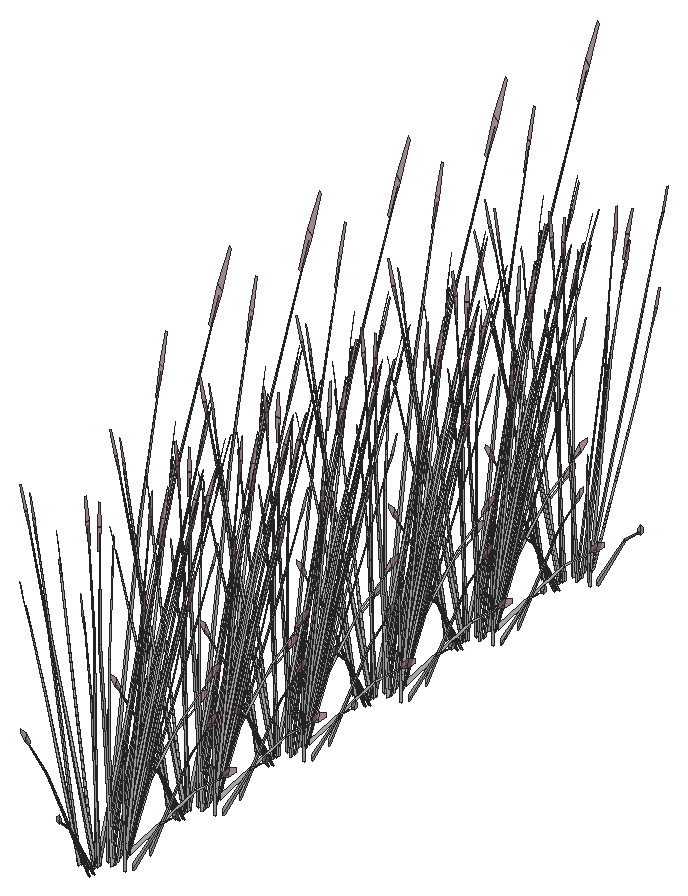
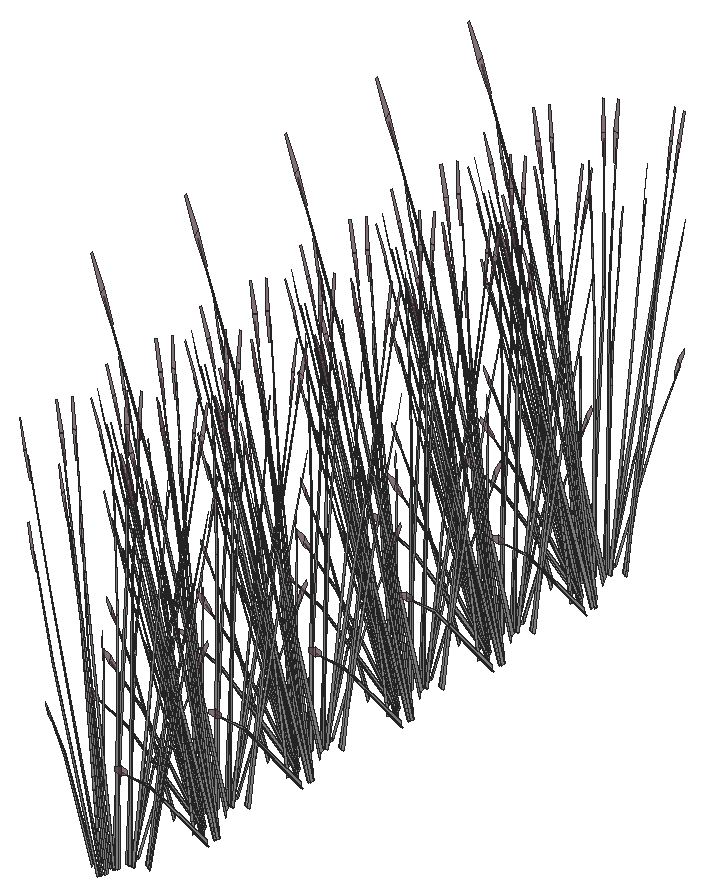
# SketchUp Ruby script. Lengths in inches.
U = 1.inch
M = Sketchup.active_model
def pt(a) = Geom::Point3d.new(a.map { |v| v * U })
def face(e, loops, mat)
  f = e.add_face(loops[0].map { |a| pt(a) })
  loops[1..].each { |l| e.add_face(l.map { |a| pt(a) }).erase! }
  f.material = f.back_material = mat if mat
  f
end
# faces: each face lists its corners as indices into pts; further lists are holes
def faces(e, pts, list, mat = nil) = list.each { |f| face(e, (f[0].is_a?(Array) ? f : [f]).map { |l| l.map { |i| pts[i] } }, mat) }
# xy, xz, yz: faces in a plane at the given z, y or x. An outline is a flat list of corners, or four numbers for a rectangle; further outlines are holes
def ring(l) = l.size == 4 ? [[l[0], l[1]], [l[2], l[1]], [l[2], l[3]], [l[0], l[3]]] : l.each_slice(2).to_a
def flat(e, list, mat, &to3) = list.each { |f| face(e, (f[0].is_a?(Array) ? f : [f]).map { |l| ring(l).map { |u, v| to3.(u, v) } }, mat) }
def xy(e, z, list, mat = nil) = flat(e, list, mat) { |x, y| [x, y, z] }
def xz(e, y, list, mat = nil) = flat(e, list, mat) { |x, z| [x, y, z] }
def yz(e, x, list, mat = nil) = flat(e, list, mat) { |y, z| [x, y, z] }
def lines(e, pts, list) = list.each { |a, b| e.add_line(pt(pts[a]), pt(pts[b])) }
# prism: a flat outline (further loops are holes) pulled along v
def prism(e, loops, v, mat = nil)
  f = face(e, loops, mat); d = Geom::Vector3d.new(v.map { |x| x * U })
  f.pushpull(f.normal.samedirection?(d) ? d.length : -d.length)
end
def box(e, o, s, mat = nil) = prism(e, [[o, [o[0] + s[0], o[1], o[2]], [o[0] + s[0], o[1] + s[1], o[2]], [o[0], o[1] + s[1], o[2]]]], [0, 0, s[2]], mat)
def at(x, y, z, deg = 0) = Geom::Transformation.translation(pt([x, y, z])) * Geom::Transformation.rotation(ORIGIN, Z_AXIS, deg.degrees)
def axes(o, x, y, z) = Geom::Transformation.new([*x, 0, *y, 0, *z, 0, *pt(o).to_a, 1])
def part(name) = M.definitions.add(name)
# library, detail: a bought-in or finely detailed component or shape, given as its bounding box
def library(name, o, s) = part(name).tap { |d| box(d.entities, o, s) }
def detail(e, o, s) = box(e.add_group.entities, o, s)
def put(e, d, t, mat = nil) = e.add_instance(d, t).tap { |i| i.material = mat if mat }
def group(e, t, mat = nil) = e.add_group.tap { |g| g.transformation = t; g.material = mat if mat }.entities
root = M.entities
M.materials.add("LightPink_Translucent").color = [144, 107, 117]
M.materials["LightPink_Translucent"].alpha = 0.75
M.materials.add("[_0053_Ivory_]").color = [200, 200, 200]
c1 = part("blade")
p = [[2.15,0.21,22],[0,0.17,0],[0.09,0.45,0],[2.18,0.31,22],[2.29,0.31,22],[0.38,0.45,0],
  [2.48,0.24,33],[2.49,0.24,33],[2.48,0.22,33]]
faces(c1.entities,p,[[0,1,2,3],[4,5,2,3],[6,3,4,7],[8,0,3,6]])
c2 = part("seeds")
p = [[0.3,-0.1,1.38],[-0.01,-0.03,1.59],[-0.01,-0.03,0.03],[0.14,-0.07,-0.07],[0.29,-0.03,3],[0.15,0.01,3.11]]
faces(c2.entities,p,[[0,1,2,3],[1,0,4,5]],"LightPink_Translucent")
c3 = part("blade with seeds")
put(c3.entities,c1,at(0,0,0))
put(c3.entities,c2,axes([2.4,0.25,30.99],[1.5799,-0.05474,1.17369],[-0.12525,1.92788,0.29478],[-0.07173,-0.02425,1.56792]))
put(root,c3,axes([680.31,309.62,38.7],[-0.1831,0.48359,0.35414],[-0.53419,-0.14105,-0.4572],[-0.04898,-0.1947,0.87481]),"[_0053_Ivory_]")
put(root,c3,axes([679.33,257.15,38.72],[-0.59846,-0.1644,0.53283],[0.20464,-0.54049,0.43934],[0.03596,0.21255,1.10256]),"[_0053_Ivory_]")
put(root,c3,axes([679.33,268.3,38.72],[-0.59846,-0.1644,0.53283],[0.20464,-0.54049,0.43934],[0.03596,0.21255,1.10256]),"[_0053_Ivory_]")
put(root,c3,axes([679.33,279.29,38.72],[-0.59846,-0.1644,0.53283],[0.20464,-0.54049,0.43934],[0.03596,0.21255,1.10256]),"[_0053_Ivory_]")
put(root,c3,axes([679.33,291.34,38.72],[-0.59846,-0.1644,0.53283],[0.20464,-0.54049,0.43934],[0.03596,0.21255,1.10256]),"[_0053_Ivory_]")
put(root,c3,axes([679.33,302.71,38.72],[-0.59846,-0.1644,0.53283],[0.20464,-0.54049,0.43934],[0.03596,0.21255,1.10256]),"[_0053_Ivory_]")
put(root,c3,axes([679.18,257.2,38.38],[-0.44753,0.21372,0.0643],[-0.21905,-0.38973,0.50621],[0.04322,0.1718,0.77189]),"[_0053_Ivory_]")
put(root,c3,axes([679.18,268.34,38.38],[-0.44753,0.21372,0.0643],[-0.21905,-0.38973,0.50621],[0.04322,0.1718,0.77189]),"[_0053_Ivory_]")
put(root,c3,axes([679.18,279.34,38.38],[-0.44753,0.21372,0.0643],[-0.21905,-0.38973,0.50621],[0.04322,0.1718,0.77189]),"[_0053_Ivory_]")
put(root,c3,axes([679.18,291.38,38.38],[-0.44753,0.21372,0.0643],[-0.21905,-0.38973,0.50621],[0.04322,0.1718,0.77189]),"[_0053_Ivory_]")
put(root,c3,axes([679.18,302.75,38.38],[-0.44753,0.21372,0.0643],[-0.21905,-0.38973,0.50621],[0.04322,0.1718,0.77189]),"[_0053_Ivory_]")
put(root,c3,axes([680.48,251.65,38.38],[0.44753,-0.21372,0.0643],[0.21905,0.38973,0.50621],[-0.04322,-0.1718,0.77189]),"[_0053_Ivory_]")
put(root,c3,axes([680.48,262.8,38.38],[0.44753,-0.21372,0.0643],[0.21905,0.38973,0.50621],[-0.04322,-0.1718,0.77189]),"[_0053_Ivory_]")
put(root,c3,axes([680.48,273.79,38.38],[0.44753,-0.21372,0.0643],[0.21905,0.38973,0.50621],[-0.04322,-0.1718,0.77189]),"[_0053_Ivory_]")
put(root,c3,axes([680.48,285.84,38.38],[0.44753,-0.21372,0.0643],[0.21905,0.38973,0.50621],[-0.04322,-0.1718,0.77189]),"[_0053_Ivory_]")
put(root,c3,axes([680.48,297.2,38.38],[0.44753,-0.21372,0.0643],[0.21905,0.38973,0.50621],[-0.04322,-0.1718,0.77189]),"[_0053_Ivory_]")
put(root,c3,axes([680.48,309.18,38.38],[0.44753,-0.21372,0.0643],[0.21905,0.38973,0.50621],[-0.04322,-0.1718,0.77189]),"[_0053_Ivory_]")
put(root,c3,axes([679.02,258.125,38.37],[0.07699,0.10127,1.74944],[0.6213,0.03978,-0.27667],[0.06248,0.22333,0.14031]),"[_0053_Ivory_]")
put(root,c3,axes([679.02,269.27,38.37],[0.07699,0.10127,1.74944],[0.6213,0.03978,-0.27667],[0.06248,0.22333,0.14031]),"[_0053_Ivory_]")
put(root,c3,axes([679.02,280.26,38.37],[0.07699,0.10127,1.74944],[0.6213,0.03978,-0.27667],[0.06248,0.22333,0.14031]),"[_0053_Ivory_]")
put(root,c3,axes([679.02,292.31,38.37],[0.07699,0.10127,1.74944],[0.6213,0.03978,-0.27667],[0.06248,0.22333,0.14031]),"[_0053_Ivory_]")
put(root,c3,axes([679.02,303.67,38.37],[0.07699,0.10127,1.74944],[0.6213,0.03978,-0.27667],[0.06248,0.22333,0.14031]),"[_0053_Ivory_]")
put(root,c3,axes([680.32,251.7,38.39],[0.59846,0.1644,0.48003],[-0.20464,0.54049,0.3958],[-0.03596,-0.21255,0.9933]),"[_0053_Ivory_]")
put(root,c3,axes([680.32,262.84,38.39],[0.59846,0.1644,0.48003],[-0.20464,0.54049,0.3958],[-0.03596,-0.21255,0.9933]),"[_0053_Ivory_]")
put(root,c3,axes([680.32,273.83,38.39],[0.59846,0.1644,0.48003],[-0.20464,0.54049,0.3958],[-0.03596,-0.21255,0.9933]),"[_0053_Ivory_]")
put(root,c3,axes([680.32,285.88,38.39],[0.59846,0.1644,0.48003],[-0.20464,0.54049,0.3958],[-0.03596,-0.21255,0.9933]),"[_0053_Ivory_]")
put(root,c3,axes([680.32,297.25,38.39],[0.59846,0.1644,0.48003],[-0.20464,0.54049,0.3958],[-0.03596,-0.21255,0.9933]),"[_0053_Ivory_]")
put(root,c3,axes([680.32,309.22,38.39],[0.59846,0.1644,0.48003],[-0.20464,0.54049,0.3958],[-0.03596,-0.21255,0.9933]),"[_0053_Ivory_]")
put(root,c3,axes([679.34,256.76,38.7],[0.1831,-0.48359,0.35414],[0.53419,0.14105,-0.4572],[0.04898,0.1947,0.87481]),"[_0053_Ivory_]")
put(root,c3,axes([679.34,267.91,38.7],[0.1831,-0.48359,0.35414],[0.53419,0.14105,-0.4572],[0.04898,0.1947,0.87481]),"[_0053_Ivory_]")
put(root,c3,axes([679.34,278.9,38.7],[0.1831,-0.48359,0.35414],[0.53419,0.14105,-0.4572],[0.04898,0.1947,0.87481]),"[_0053_Ivory_]")
put(root,c3,axes([679.34,290.94,38.7],[0.1831,-0.48359,0.35414],[0.53419,0.14105,-0.4572],[0.04898,0.1947,0.87481]),"[_0053_Ivory_]")
put(root,c3,axes([679.34,302.31,38.7],[0.1831,-0.48359,0.35414],[0.53419,0.14105,-0.4572],[0.04898,0.1947,0.87481]),"[_0053_Ivory_]")
put(root,c3,axes([680.06,258.48,39.3],[0.4197,-0.36076,-0.06488],[0.38456,0.39511,-0.29416],[0.02707,0.11196,0.97024]),"[_0053_Ivory_]")
put(root,c3,axes([680.06,269.63,39.3],[0.4197,-0.36076,-0.06488],[0.38456,0.39511,-0.29416],[0.02707,0.11196,0.97024]),"[_0053_Ivory_]")
put(root,c3,axes([680.06,280.62,39.3],[0.4197,-0.36076,-0.06488],[0.38456,0.39511,-0.29416],[0.02707,0.11196,0.97024]),"[_0053_Ivory_]")
put(root,c3,axes([680.06,292.67,39.3],[0.4197,-0.36076,-0.06488],[0.38456,0.39511,-0.29416],[0.02707,0.11196,0.97024]),"[_0053_Ivory_]")
put(root,c3,axes([680.06,304.03,39.3],[0.4197,-0.36076,-0.06488],[0.38456,0.39511,-0.29416],[0.02707,0.11196,0.97024]),"[_0053_Ivory_]")
put(root,c3,axes([679.16,256.96,38.6875],[0.59433,-0.29278,-0.1216],[0.29207,0.51964,-0.67495],[0.07842,0.21898,1.02557]),"[_0053_Ivory_]")
put(root,c3,axes([679.16,268.11,38.6875],[0.59433,-0.29278,-0.1216],[0.29207,0.51964,-0.67495],[0.07842,0.21898,1.02557]),"[_0053_Ivory_]")
put(root,c3,axes([679.16,279.1,38.6875],[0.59433,-0.29278,-0.1216],[0.29207,0.51964,-0.67495],[0.07842,0.21898,1.02557]),"[_0053_Ivory_]")
put(root,c3,axes([679.16,291.14,38.6875],[0.59433,-0.29278,-0.1216],[0.29207,0.51964,-0.67495],[0.07842,0.21898,1.02557]),"[_0053_Ivory_]")
put(root,c3,axes([679.16,302.51,38.6875],[0.59433,-0.29278,-0.1216],[0.29207,0.51964,-0.67495],[0.07842,0.21898,1.02557]),"[_0053_Ivory_]")
put(root,c3,axes([682.2,251.16,38.36],[-0.06168,0.04803,1.77383],[-0.60432,-0.16205,-0.16761],[-0.02188,-0.20961,0.31391]),"[_0053_Ivory_]")
put(root,c3,axes([682.2,262.31,38.36],[-0.06168,0.04803,1.77383],[-0.60432,-0.16205,-0.16761],[-0.02188,-0.20961,0.31391]),"[_0053_Ivory_]")
put(root,c3,axes([682.2,273.3,38.36],[-0.06168,0.04803,1.77383],[-0.60432,-0.16205,-0.16761],[-0.02188,-0.20961,0.31391]),"[_0053_Ivory_]")
put(root,c3,axes([682.2,285.34,38.36],[-0.06168,0.04803,1.77383],[-0.60432,-0.16205,-0.16761],[-0.02188,-0.20961,0.31391]),"[_0053_Ivory_]")
put(root,c3,axes([682.2,296.71,38.36],[-0.06168,0.04803,1.77383],[-0.60432,-0.16205,-0.16761],[-0.02188,-0.20961,0.31391]),"[_0053_Ivory_]")
put(root,c3,axes([682.2,308.6875,38.36],[-0.06168,0.04803,1.77383],[-0.60432,-0.16205,-0.16761],[-0.02188,-0.20961,0.31391]),"[_0053_Ivory_]")
put(root,c3,axes([681.72,252.55,38.6875],[-0.6675,-0.03116,-0.1216],[0.01824,-0.58993,-0.67495],[0.04637,-0.2272,1.02557]),"[_0053_Ivory_]")
put(root,c3,axes([681.72,263.69,38.6875],[-0.6675,-0.03116,-0.1216],[0.01824,-0.58993,-0.67495],[0.04637,-0.2272,1.02557]),"[_0053_Ivory_]")
put(root,c3,axes([681.72,274.6875,38.6875],[-0.6675,-0.03116,-0.1216],[0.01824,-0.58993,-0.67495],[0.04637,-0.2272,1.02557]),"[_0053_Ivory_]")
put(root,c3,axes([681.72,286.73,38.6875],[-0.6675,-0.03116,-0.1216],[0.01824,-0.58993,-0.67495],[0.04637,-0.2272,1.02557]),"[_0053_Ivory_]")
put(root,c3,axes([681.72,298.1,38.6875],[-0.6675,-0.03116,-0.1216],[0.01824,-0.58993,-0.67495],[0.04637,-0.2272,1.02557]),"[_0053_Ivory_]")
put(root,c3,axes([681.72,310.07,38.6875],[-0.6675,-0.03116,-0.1216],[0.01824,-0.58993,-0.67495],[0.04637,-0.2272,1.02557]),"[_0053_Ivory_]")
put(root,c3,axes([681.46,252.64,38.7],[-0.41095,0.33109,0.35414],[-0.38901,-0.37805,-0.4572],[0.05919,-0.19208,0.87481]),"[_0053_Ivory_]")
put(root,c3,axes([681.46,263.79,38.7],[-0.41095,0.33109,0.35414],[-0.38901,-0.37805,-0.4572],[0.05919,-0.19208,0.87481]),"[_0053_Ivory_]")
put(root,c3,axes([681.46,274.78,38.7],[-0.41095,0.33109,0.35414],[-0.38901,-0.37805,-0.4572],[0.05919,-0.19208,0.87481]),"[_0053_Ivory_]")
put(root,c3,axes([681.46,286.82,38.7],[-0.41095,0.33109,0.35414],[-0.38901,-0.37805,-0.4572],[0.05919,-0.19208,0.87481]),"[_0053_Ivory_]")
put(root,c3,axes([681.46,298.1875,38.7],[-0.41095,0.33109,0.35414],[-0.38901,-0.37805,-0.4572],[0.05919,-0.19208,0.87481]),"[_0053_Ivory_]")
put(root,c3,axes([681.46,310.17,38.7],[-0.41095,0.33109,0.35414],[-0.38901,-0.37805,-0.4572],[0.05919,-0.19208,0.87481]),"[_0053_Ivory_]")
put(root,c3,axes([680.82,257.02,38.39],[-0.60408,0.14432,0.48003],[-0.10484,-0.56611,0.3958],[0.14207,0.16684,0.9933]),"[_0053_Ivory_]")
put(root,c3,axes([680.82,268.17,38.39],[-0.60408,0.14432,0.48003],[-0.10484,-0.56611,0.3958],[0.14207,0.16684,0.9933]),"[_0053_Ivory_]")
put(root,c3,axes([680.82,279.16,38.39],[-0.60408,0.14432,0.48003],[-0.10484,-0.56611,0.3958],[0.14207,0.16684,0.9933]),"[_0053_Ivory_]")
put(root,c3,axes([680.82,291.21,38.39],[-0.60408,0.14432,0.48003],[-0.10484,-0.56611,0.3958],[0.14207,0.16684,0.9933]),"[_0053_Ivory_]")
put(root,c3,axes([680.82,302.58,38.39],[-0.60408,0.14432,0.48003],[-0.10484,-0.56611,0.3958],[0.14207,0.16684,0.9933]),"[_0053_Ivory_]")
put(root,c3,axes([680.71,257.14,38.38],[-0.27604,0.39948,0.0643],[-0.39309,-0.23258,0.50621],[0.12709,0.12808,0.77189]),"[_0053_Ivory_]")
put(root,c3,axes([680.71,268.28,38.38],[-0.27604,0.39948,0.0643],[-0.39309,-0.23258,0.50621],[0.12709,0.12808,0.77189]),"[_0053_Ivory_]")
put(root,c3,axes([680.71,279.28,38.38],[-0.27604,0.39948,0.0643],[-0.39309,-0.23258,0.50621],[0.12709,0.12808,0.77189]),"[_0053_Ivory_]")
put(root,c3,axes([680.71,291.32,38.38],[-0.27604,0.39948,0.0643],[-0.39309,-0.23258,0.50621],[0.12709,0.12808,0.77189]),"[_0053_Ivory_]")
put(root,c3,axes([680.71,302.6875,38.38],[-0.27604,0.39948,0.0643],[-0.39309,-0.23258,0.50621],[0.12709,0.12808,0.77189]),"[_0053_Ivory_]")
put(root,c3,axes([680.625,256.68,38.7],[-0.0938,-0.50652,0.35414],[0.53623,-0.13375,-0.4572],[0.14403,0.14515,0.87481]),"[_0053_Ivory_]")
put(root,c3,axes([680.625,267.83,38.7],[-0.0938,-0.50652,0.35414],[0.53623,-0.13375,-0.4572],[0.14403,0.14515,0.87481]),"[_0053_Ivory_]")
put(root,c3,axes([680.625,278.82,38.7],[-0.0938,-0.50652,0.35414],[0.53623,-0.13375,-0.4572],[0.14403,0.14515,0.87481]),"[_0053_Ivory_]")
put(root,c3,axes([680.625,290.86,38.7],[-0.0938,-0.50652,0.35414],[0.53623,-0.13375,-0.4572],[0.14403,0.14515,0.87481]),"[_0053_Ivory_]")
put(root,c3,axes([680.625,302.23,38.7],[-0.0938,-0.50652,0.35414],[0.53623,-0.13375,-0.4572],[0.14403,0.14515,0.87481]),"[_0053_Ivory_]")
put(root,c3,axes([680.98,253.76,38.13],[-0.52482,-0.32674,1.38283],[0.55416,-0.50872,0.59665],[0.16933,0.30658,1.33663]),"[_0053_Ivory_]")
put(root,c3,axes([680.98,264.91,38.13],[-0.52482,-0.32674,1.38283],[0.55416,-0.50872,0.59665],[0.16933,0.30658,1.33663]),"[_0053_Ivory_]")
put(root,c3,axes([680.98,275.9,38.13],[-0.52482,-0.32674,1.38283],[0.55416,-0.50872,0.59665],[0.16933,0.30658,1.33663]),"[_0053_Ivory_]")
put(root,c3,axes([680.98,287.95,38.13],[-0.52482,-0.32674,1.38283],[0.55416,-0.50872,0.59665],[0.16933,0.30658,1.33663]),"[_0053_Ivory_]")
put(root,c3,axes([680.98,299.3125,38.13],[-0.52482,-0.32674,1.38283],[0.55416,-0.50872,0.59665],[0.16933,0.30658,1.33663]),"[_0053_Ivory_]")
put(root,c3,axes([680.1,257.39,38.36],[0.0018,-0.07613,1.77383],[0.52048,-0.3359,-0.16761],[0.18079,0.11989,0.31391]),"[_0053_Ivory_]")
put(root,c3,axes([680.1,268.53,38.36],[0.0018,-0.07613,1.77383],[0.52048,-0.3359,-0.16761],[0.18079,0.11989,0.31391]),"[_0053_Ivory_]")
put(root,c3,axes([680.1,279.53,38.36],[0.0018,-0.07613,1.77383],[0.52048,-0.3359,-0.16761],[0.18079,0.11989,0.31391]),"[_0053_Ivory_]")
put(root,c3,axes([680.1,291.57,38.36],[0.0018,-0.07613,1.77383],[0.52048,-0.3359,-0.16761],[0.18079,0.11989,0.31391]),"[_0053_Ivory_]")
put(root,c3,axes([680.1,302.9375,38.36],[0.0018,-0.07613,1.77383],[0.52048,-0.3359,-0.16761],[0.18079,0.11989,0.31391]),"[_0053_Ivory_]")
put(root,c3,axes([681.84,252.34,38.38],[0.49911,0.0293,0.0643],[-0.01368,0.44245,0.50621],[0.05223,-0.16948,0.77189]),"[_0053_Ivory_]")
put(root,c3,axes([681.84,263.49,38.38],[0.49911,0.0293,0.0643],[-0.01368,0.44245,0.50621],[0.05223,-0.16948,0.77189]),"[_0053_Ivory_]")
put(root,c3,axes([681.84,274.48,38.38],[0.49911,0.0293,0.0643],[-0.01368,0.44245,0.50621],[0.05223,-0.16948,0.77189]),"[_0053_Ivory_]")
put(root,c3,axes([681.84,286.52,38.38],[0.49911,0.0293,0.0643],[-0.01368,0.44245,0.50621],[0.05223,-0.16948,0.77189]),"[_0053_Ivory_]")
put(root,c3,axes([681.84,297.89,38.38],[0.49911,0.0293,0.0643],[-0.01368,0.44245,0.50621],[0.05223,-0.16948,0.77189]),"[_0053_Ivory_]")
put(root,c3,axes([681.84,309.86,38.38],[0.49911,0.0293,0.0643],[-0.01368,0.44245,0.50621],[0.05223,-0.16948,0.77189]),"[_0053_Ivory_]")
put(root,c3,axes([682.33,251.61,38.37],[-0.00586,-0.12516,1.74944],[-0.49517,-0.36172,-0.27667],[0.07656,-0.21927,0.14031]),"[_0053_Ivory_]")
put(root,c3,axes([682.33,262.76,38.37],[-0.00586,-0.12516,1.74944],[-0.49517,-0.36172,-0.27667],[0.07656,-0.21927,0.14031]),"[_0053_Ivory_]")
put(root,c3,axes([682.33,273.75,38.37],[-0.00586,-0.12516,1.74944],[-0.49517,-0.36172,-0.27667],[0.07656,-0.21927,0.14031]),"[_0053_Ivory_]")
put(root,c3,axes([682.33,285.79,38.37],[-0.00586,-0.12516,1.74944],[-0.49517,-0.36172,-0.27667],[0.07656,-0.21927,0.14031]),"[_0053_Ivory_]")
put(root,c3,axes([682.33,297.16,38.37],[-0.00586,-0.12516,1.74944],[-0.49517,-0.36172,-0.27667],[0.07656,-0.21927,0.14031]),"[_0053_Ivory_]")
put(root,c3,axes([682.33,309.14,38.37],[-0.00586,-0.12516,1.74944],[-0.49517,-0.36172,-0.27667],[0.07656,-0.21927,0.14031]),"[_0053_Ivory_]")
put(root,c3,axes([681.68,252.3,38.39],[0.43249,0.42907,0.48003],[-0.45929,0.37004,0.3958],[0.07978,-0.2013,0.9933]),"[_0053_Ivory_]")
put(root,c3,axes([681.68,263.44,38.39],[0.43249,0.42907,0.48003],[-0.45929,0.37004,0.3958],[0.07978,-0.2013,0.9933]),"[_0053_Ivory_]")
put(root,c3,axes([681.68,274.4375,38.39],[0.43249,0.42907,0.48003],[-0.45929,0.37004,0.3958],[0.07978,-0.2013,0.9933]),"[_0053_Ivory_]")
put(root,c3,axes([681.68,286.48,38.39],[0.43249,0.42907,0.48003],[-0.45929,0.37004,0.3958],[0.07978,-0.2013,0.9933]),"[_0053_Ivory_]")
put(root,c3,axes([681.68,297.85,38.39],[0.43249,0.42907,0.48003],[-0.45929,0.37004,0.3958],[0.07978,-0.2013,0.9933]),"[_0053_Ivory_]")
put(root,c3,axes([681.68,309.82,38.39],[0.43249,0.42907,0.48003],[-0.45929,0.37004,0.3958],[0.07978,-0.2013,0.9933]),"[_0053_Ivory_]")
put(root,c3,axes([682.18,253.66,38.7],[-0.52868,0.08987,0.35414],[-0.1396,-0.51376,-0.4572],[0.1515,-0.13799,0.87481]),"[_0053_Ivory_]")
put(root,c3,axes([682.18,264.81,38.7],[-0.52868,0.08987,0.35414],[-0.1396,-0.51376,-0.4572],[0.1515,-0.13799,0.87481]),"[_0053_Ivory_]")
put(root,c3,axes([682.18,275.8,38.7],[-0.52868,0.08987,0.35414],[-0.1396,-0.51376,-0.4572],[0.1515,-0.13799,0.87481]),"[_0053_Ivory_]")
put(root,c3,axes([682.18,287.84,38.7],[-0.52868,0.08987,0.35414],[-0.1396,-0.51376,-0.4572],[0.1515,-0.13799,0.87481]),"[_0053_Ivory_]")
put(root,c3,axes([682.18,299.21,38.7],[-0.52868,0.08987,0.35414],[-0.1396,-0.51376,-0.4572],[0.1515,-0.13799,0.87481]),"[_0053_Ivory_]")
put(root,c3,axes([682.18,311.1875,38.7],[-0.52868,0.08987,0.35414],[-0.1396,-0.51376,-0.4572],[0.1515,-0.13799,0.87481]),"[_0053_Ivory_]")
put(root,c3,axes([680.57,256.9375,38.6875],[0.36191,-0.53827,-0.1216],[0.52412,0.3101,-0.67495],[0.18219,0.15207,1.02557]),"[_0053_Ivory_]")
put(root,c3,axes([680.57,268.09,38.6875],[0.36191,-0.53827,-0.1216],[0.52412,0.3101,-0.67495],[0.18219,0.15207,1.02557]),"[_0053_Ivory_]")
put(root,c3,axes([680.57,279.08,38.6875],[0.36191,-0.53827,-0.1216],[0.52412,0.3101,-0.67495],[0.18219,0.15207,1.02557]),"[_0053_Ivory_]")
put(root,c3,axes([680.57,291.12,38.6875],[0.36191,-0.53827,-0.1216],[0.52412,0.3101,-0.67495],[0.18219,0.15207,1.02557]),"[_0053_Ivory_]")
put(root,c3,axes([680.57,302.49,38.6875],[0.36191,-0.53827,-0.1216],[0.52412,0.3101,-0.67495],[0.18219,0.15207,1.02557]),"[_0053_Ivory_]")
put(root,c3,axes([682.45,253.71,38.6875],[-0.56181,-0.34675,-0.1216],[0.32367,-0.50216,-0.67495],[0.15873,-0.17455,1.02557]),"[_0053_Ivory_]")
put(root,c3,axes([682.45,264.86,38.6875],[-0.56181,-0.34675,-0.1216],[0.32367,-0.50216,-0.67495],[0.15873,-0.17455,1.02557]),"[_0053_Ivory_]")
put(root,c3,axes([682.45,275.85,38.6875],[-0.56181,-0.34675,-0.1216],[0.32367,-0.50216,-0.67495],[0.15873,-0.17455,1.02557]),"[_0053_Ivory_]")
put(root,c3,axes([682.45,287.89,38.6875],[-0.56181,-0.34675,-0.1216],[0.32367,-0.50216,-0.67495],[0.15873,-0.17455,1.02557]),"[_0053_Ivory_]")
put(root,c3,axes([682.45,299.26,38.6875],[-0.56181,-0.34675,-0.1216],[0.32367,-0.50216,-0.67495],[0.15873,-0.17455,1.02557]),"[_0053_Ivory_]")
put(root,c3,axes([682.45,311.24,38.6875],[-0.56181,-0.34675,-0.1216],[0.32367,-0.50216,-0.67495],[0.15873,-0.17455,1.02557]),"[_0053_Ivory_]")
put(root,c3,axes([681.69,255.99,38.7],[-0.34557,-0.39372,0.35414],[0.39459,-0.37271,-0.4572],[0.20048,0.05671,0.87481]),"[_0053_Ivory_]")
put(root,c3,axes([681.69,267.14,38.7],[-0.34557,-0.39372,0.35414],[0.39459,-0.37271,-0.4572],[0.20048,0.05671,0.87481]),"[_0053_Ivory_]")
put(root,c3,axes([681.69,278.13,38.7],[-0.34557,-0.39372,0.35414],[0.39459,-0.37271,-0.4572],[0.20048,0.05671,0.87481]),"[_0053_Ivory_]")
put(root,c3,axes([681.69,290.18,38.7],[-0.34557,-0.39372,0.35414],[0.39459,-0.37271,-0.4572],[0.20048,0.05671,0.87481]),"[_0053_Ivory_]")
put(root,c3,axes([681.69,301.54,38.7],[-0.34557,-0.39372,0.35414],[0.39459,-0.37271,-0.4572],[0.20048,0.05671,0.87481]),"[_0053_Ivory_]")
put(root,c3,axes([682.01,256.35,38.38],[-0.03058,0.47819,0.0643],[-0.4618,-0.01311,0.50621],[0.1769,0.05004,0.77189]),"[_0053_Ivory_]")
put(root,c3,axes([682.01,267.5,38.38],[-0.03058,0.47819,0.0643],[-0.4618,-0.01311,0.50621],[0.1769,0.05004,0.77189]),"[_0053_Ivory_]")
put(root,c3,axes([682.01,278.49,38.38],[-0.03058,0.47819,0.0643],[-0.4618,-0.01311,0.50621],[0.1769,0.05004,0.77189]),"[_0053_Ivory_]")
put(root,c3,axes([682.01,290.53,38.38],[-0.03058,0.47819,0.0643],[-0.4618,-0.01311,0.50621],[0.1769,0.05004,0.77189]),"[_0053_Ivory_]")
put(root,c3,axes([682.01,301.9,38.38],[-0.03058,0.47819,0.0643],[-0.4618,-0.01311,0.50621],[0.1769,0.05004,0.77189]),"[_0053_Ivory_]")
put(root,c3,axes([682.05,256.2,38.39],[-0.44783,0.41436,0.48003],[-0.38623,-0.44004,0.3958],[0.21011,0.07643,0.9933]),"[_0053_Ivory_]")
put(root,c3,axes([682.05,267.35,38.39],[-0.44783,0.41436,0.48003],[-0.38623,-0.44004,0.3958],[0.21011,0.07643,0.9933]),"[_0053_Ivory_]")
put(root,c3,axes([682.05,278.34,38.39],[-0.44783,0.41436,0.48003],[-0.38623,-0.44004,0.3958],[0.21011,0.07643,0.9933]),"[_0053_Ivory_]")
put(root,c3,axes([682.05,290.38,38.39],[-0.44783,0.41436,0.48003],[-0.38623,-0.44004,0.3958],[0.21011,0.07643,0.9933]),"[_0053_Ivory_]")
put(root,c3,axes([682.05,301.75,38.39],[-0.44783,0.41436,0.48003],[-0.38623,-0.44004,0.3958],[0.21011,0.07643,0.9933]),"[_0053_Ivory_]")
put(root,c3,axes([682.26,254.89,38.7],[-0.50475,-0.17543,0.35414],[0.14722,-0.5118,-0.4572],[0.20322,-0.04693,0.87481]),"[_0053_Ivory_]")
put(root,c3,axes([682.26,266.04,38.7],[-0.50475,-0.17543,0.35414],[0.14722,-0.5118,-0.4572],[0.20322,-0.04693,0.87481]),"[_0053_Ivory_]")
put(root,c3,axes([682.26,277.03,38.7],[-0.50475,-0.17543,0.35414],[0.14722,-0.5118,-0.4572],[0.20322,-0.04693,0.87481]),"[_0053_Ivory_]")
put(root,c3,axes([682.26,289.07,38.7],[-0.50475,-0.17543,0.35414],[0.14722,-0.5118,-0.4572],[0.20322,-0.04693,0.87481]),"[_0053_Ivory_]")
put(root,c3,axes([682.26,300.44,38.7],[-0.50475,-0.17543,0.35414],[0.14722,-0.5118,-0.4572],[0.20322,-0.04693,0.87481]),"[_0053_Ivory_]")
put(root,c3,axes([682.26,312.42,38.7],[-0.50475,-0.17543,0.35414],[0.14722,-0.5118,-0.4572],[0.20322,-0.04693,0.87481]),"[_0053_Ivory_]")
put(root,c3,axes([682.66,253.58,38.38],[0.41695,0.26447,0.0643],[-0.24275,0.37662,0.50621],[0.13368,-0.12176,0.77189]),"[_0053_Ivory_]")
put(root,c3,axes([682.66,264.73,38.38],[0.41695,0.26447,0.0643],[-0.24275,0.37662,0.50621],[0.13368,-0.12176,0.77189]),"[_0053_Ivory_]")
put(root,c3,axes([682.66,275.72,38.38],[0.41695,0.26447,0.0643],[-0.24275,0.37662,0.50621],[0.13368,-0.12176,0.77189]),"[_0053_Ivory_]")
put(root,c3,axes([682.66,287.76,38.38],[0.41695,0.26447,0.0643],[-0.24275,0.37662,0.50621],[0.13368,-0.12176,0.77189]),"[_0053_Ivory_]")
put(root,c3,axes([682.66,299.13,38.38],[0.41695,0.26447,0.0643],[-0.24275,0.37662,0.50621],[0.13368,-0.12176,0.77189]),"[_0053_Ivory_]")
put(root,c3,axes([682.66,311.11,38.38],[0.41695,0.26447,0.0643],[-0.24275,0.37662,0.50621],[0.13368,-0.12176,0.77189]),"[_0053_Ivory_]")
put(root,c3,axes([682.54,253.47,38.39],[0.15063,0.57876,0.48003],[-0.59087,0.10045,0.3958],[0.17414,-0.13612,0.9933]),"[_0053_Ivory_]")
put(root,c3,axes([682.54,264.62,38.39],[0.15063,0.57876,0.48003],[-0.59087,0.10045,0.3958],[0.17414,-0.13612,0.9933]),"[_0053_Ivory_]")
put(root,c3,axes([682.54,275.61,38.39],[0.15063,0.57876,0.48003],[-0.59087,0.10045,0.3958],[0.17414,-0.13612,0.9933]),"[_0053_Ivory_]")
put(root,c3,axes([682.54,287.65,38.39],[0.15063,0.57876,0.48003],[-0.59087,0.10045,0.3958],[0.17414,-0.13612,0.9933]),"[_0053_Ivory_]")
put(root,c3,axes([682.54,299.02,38.39],[0.15063,0.57876,0.48003],[-0.59087,0.10045,0.3958],[0.17414,-0.13612,0.9933]),"[_0053_Ivory_]")
put(root,c3,axes([682.54,311,38.39],[0.15063,0.57876,0.48003],[-0.59087,0.10045,0.3958],[0.17414,-0.13612,0.9933]),"[_0053_Ivory_]")
put(root,c3,axes([683.83,253.56,38.36],[-0.07933,-0.00478,1.77383],[-0.32942,-0.51175,-0.16761],[0.13229,-0.16826,0.31391]),"[_0053_Ivory_]")
put(root,c3,axes([683.83,264.71,38.36],[-0.07933,-0.00478,1.77383],[-0.32942,-0.51175,-0.16761],[0.13229,-0.16826,0.31391]),"[_0053_Ivory_]")
put(root,c3,axes([683.83,275.7,38.36],[-0.07933,-0.00478,1.77383],[-0.32942,-0.51175,-0.16761],[0.13229,-0.16826,0.31391]),"[_0053_Ivory_]")
put(root,c3,axes([683.83,287.74,38.36],[-0.07933,-0.00478,1.77383],[-0.32942,-0.51175,-0.16761],[0.13229,-0.16826,0.31391]),"[_0053_Ivory_]")
put(root,c3,axes([683.83,299.11,38.36],[-0.07933,-0.00478,1.77383],[-0.32942,-0.51175,-0.16761],[0.13229,-0.16826,0.31391]),"[_0053_Ivory_]")
put(root,c3,axes([683.83,311.09,38.36],[-0.07933,-0.00478,1.77383],[-0.32942,-0.51175,-0.16761],[0.13229,-0.16826,0.31391]),"[_0053_Ivory_]")
put(root,c3,axes([682.72,255.05,38.38],[0.22307,0.42878,0.0643],[-0.40677,0.20987,0.50621],[0.17931,-0.04141,0.77189]),"[_0053_Ivory_]")
put(root,c3,axes([682.72,266.2,38.38],[0.22307,0.42878,0.0643],[-0.40677,0.20987,0.50621],[0.17931,-0.04141,0.77189]),"[_0053_Ivory_]")
put(root,c3,axes([682.72,277.1875,38.38],[0.22307,0.42878,0.0643],[-0.40677,0.20987,0.50621],[0.17931,-0.04141,0.77189]),"[_0053_Ivory_]")
put(root,c3,axes([682.72,289.23,38.38],[0.22307,0.42878,0.0643],[-0.40677,0.20987,0.50621],[0.17931,-0.04141,0.77189]),"[_0053_Ivory_]")
put(root,c3,axes([682.72,300.6,38.38],[0.22307,0.42878,0.0643],[-0.40677,0.20987,0.50621],[0.17931,-0.04141,0.77189]),"[_0053_Ivory_]")
put(root,c3,axes([682.72,312.58,38.38],[0.22307,0.42878,0.0643],[-0.40677,0.20987,0.50621],[0.17931,-0.04141,0.77189]),"[_0053_Ivory_]")
put(root,c3,axes([681.79,256.24,38.6875],[0.03252,-0.63953,-0.1216],[0.61574,0.01748,-0.67495],[0.23714,0.04442,1.02557]),"[_0053_Ivory_]")
put(root,c3,axes([681.79,267.39,38.6875],[0.03252,-0.63953,-0.1216],[0.61574,0.01748,-0.67495],[0.23714,0.04442,1.02557]),"[_0053_Ivory_]")
put(root,c3,axes([681.79,278.38,38.6875],[0.03252,-0.63953,-0.1216],[0.61574,0.01748,-0.67495],[0.23714,0.04442,1.02557]),"[_0053_Ivory_]")
put(root,c3,axes([681.79,290.43,38.6875],[0.03252,-0.63953,-0.1216],[0.61574,0.01748,-0.67495],[0.23714,0.04442,1.02557]),"[_0053_Ivory_]")
put(root,c3,axes([681.79,301.79,38.6875],[0.03252,-0.63953,-0.1216],[0.61574,0.01748,-0.67495],[0.23714,0.04442,1.02557]),"[_0053_Ivory_]")
put(root,c3,axes([682.47,255.0625,38.6875],[-0.30559,-0.56943,-0.1216],[0.54237,-0.27983,-0.67495],[0.22856,-0.07513,1.02557]),"[_0053_Ivory_]")
put(root,c3,axes([682.47,266.21,38.6875],[-0.30559,-0.56943,-0.1216],[0.54237,-0.27983,-0.67495],[0.22856,-0.07513,1.02557]),"[_0053_Ivory_]")
put(root,c3,axes([682.47,277.2,38.6875],[-0.30559,-0.56943,-0.1216],[0.54237,-0.27983,-0.67495],[0.22856,-0.07513,1.02557]),"[_0053_Ivory_]")
put(root,c3,axes([682.47,289.24,38.6875],[-0.30559,-0.56943,-0.1216],[0.54237,-0.27983,-0.67495],[0.22856,-0.07513,1.02557]),"[_0053_Ivory_]")
put(root,c3,axes([682.47,300.61,38.6875],[-0.30559,-0.56943,-0.1216],[0.54237,-0.27983,-0.67495],[0.22856,-0.07513,1.02557]),"[_0053_Ivory_]")
put(root,c3,axes([682.47,312.59,38.6875],[-0.30559,-0.56943,-0.1216],[0.54237,-0.27983,-0.67495],[0.22856,-0.07513,1.02557]),"[_0053_Ivory_]")
put(root,c3,axes([682.68,254.9,38.39],[-0.17159,0.57338,0.48003],[-0.56413,-0.19607,0.3958],[0.22185,-0.03446,0.9933]),"[_0053_Ivory_]")
put(root,c3,axes([682.68,266.04,38.39],[-0.17159,0.57338,0.48003],[-0.56413,-0.19607,0.3958],[0.22185,-0.03446,0.9933]),"[_0053_Ivory_]")
put(root,c3,axes([682.68,277.04,38.39],[-0.17159,0.57338,0.48003],[-0.56413,-0.19607,0.3958],[0.22185,-0.03446,0.9933]),"[_0053_Ivory_]")
put(root,c3,axes([682.68,289.08,38.39],[-0.17159,0.57338,0.48003],[-0.56413,-0.19607,0.3958],[0.22185,-0.03446,0.9933]),"[_0053_Ivory_]")
put(root,c3,axes([682.68,300.45,38.39],[-0.17159,0.57338,0.48003],[-0.56413,-0.19607,0.3958],[0.22185,-0.03446,0.9933]),"[_0053_Ivory_]")
put(root,c3,axes([682.68,312.42,38.39],[-0.17159,0.57338,0.48003],[-0.56413,-0.19607,0.3958],[0.22185,-0.03446,0.9933]),"[_0053_Ivory_]")
put(root,c3,axes([682.32,255.86,38.37],[0.13029,-0.01064,1.74944],[0.35737,-0.48855,-0.27667],[0.23175,0.06449,0.14031]),"[_0053_Ivory_]")
put(root,c3,axes([682.32,267.01,38.37],[0.13029,-0.01064,1.74944],[0.35737,-0.48855,-0.27667],[0.23175,0.06449,0.14031]),"[_0053_Ivory_]")
put(root,c3,axes([682.32,278,38.37],[0.13029,-0.01064,1.74944],[0.35737,-0.48855,-0.27667],[0.23175,0.06449,0.14031]),"[_0053_Ivory_]")
put(root,c3,axes([682.32,290.04,38.37],[0.13029,-0.01064,1.74944],[0.35737,-0.48855,-0.27667],[0.23175,0.06449,0.14031]),"[_0053_Ivory_]")
put(root,c3,axes([682.32,301.41,38.37],[0.13029,-0.01064,1.74944],[0.35737,-0.48855,-0.27667],[0.23175,0.06449,0.14031]),"[_0053_Ivory_]")
put(root,c3,axes([683.6875,256.75,38.36],[-0.05492,-0.05505,1.77383],[0.12013,-0.59013,-0.16761],[0.21632,-0.0377,0.31391]),"[_0053_Ivory_]")
put(root,c3,axes([683.6875,267.9,38.36],[-0.05492,-0.05505,1.77383],[0.12013,-0.59013,-0.16761],[0.21632,-0.0377,0.31391]),"[_0053_Ivory_]")
put(root,c3,axes([683.6875,278.89,38.36],[-0.05492,-0.05505,1.77383],[0.12013,-0.59013,-0.16761],[0.21632,-0.0377,0.31391]),"[_0053_Ivory_]")
put(root,c3,axes([683.6875,290.94,38.36],[-0.05492,-0.05505,1.77383],[0.12013,-0.59013,-0.16761],[0.21632,-0.0377,0.31391]),"[_0053_Ivory_]")
put(root,c3,axes([683.6875,302.3,38.36],[-0.05492,-0.05505,1.77383],[0.12013,-0.59013,-0.16761],[0.21632,-0.0377,0.31391]),"[_0053_Ivory_]")
put(root,c3,axes([684.13,254.17,38.37],[0.08428,-0.09579,1.74944],[-0.10787,-0.58756,-0.27667],[0.21147,-0.1114,0.14031]),"[_0053_Ivory_]")
put(root,c3,axes([684.13,265.32,38.37],[0.08428,-0.09579,1.74944],[-0.10787,-0.58756,-0.27667],[0.21147,-0.1114,0.14031]),"[_0053_Ivory_]")
put(root,c3,axes([684.13,276.31,38.37],[0.08428,-0.09579,1.74944],[-0.10787,-0.58756,-0.27667],[0.21147,-0.1114,0.14031]),"[_0053_Ivory_]")
put(root,c3,axes([684.13,288.35,38.37],[0.08428,-0.09579,1.74944],[-0.10787,-0.58756,-0.27667],[0.21147,-0.1114,0.14031]),"[_0053_Ivory_]")
put(root,c3,axes([684.13,299.72,38.37],[0.08428,-0.09579,1.74944],[-0.10787,-0.58756,-0.27667],[0.21147,-0.1114,0.14031]),"[_0053_Ivory_]")
put(root,c3,axes([684.13,311.7,38.37],[0.08428,-0.09579,1.74944],[-0.10787,-0.58756,-0.27667],[0.21147,-0.1114,0.14031]),"[_0053_Ivory_]")
